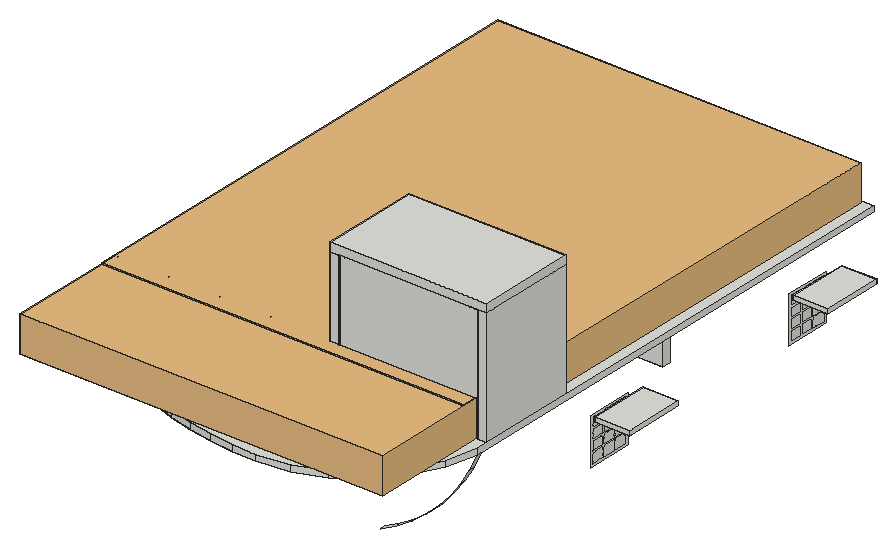
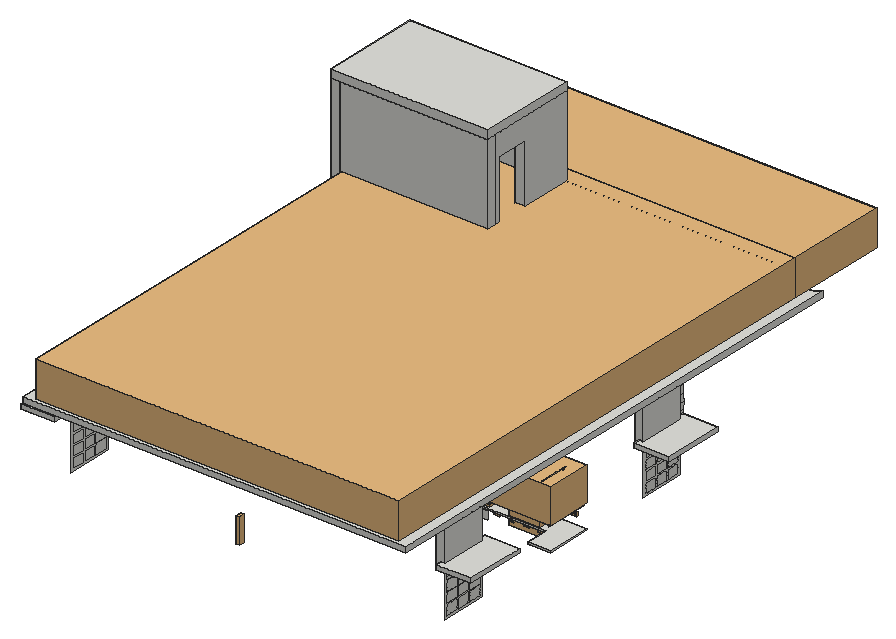
# SketchUp Ruby script. Lengths in inches.
U = 1.inch
M = Sketchup.active_model
def pt(a) = Geom::Point3d.new(a.map { |v| v * U })
def face(e, loops, mat)
  f = e.add_face(loops[0].map { |a| pt(a) })
  loops[1..].each { |l| e.add_face(l.map { |a| pt(a) }).erase! }
  f.material = f.back_material = mat if mat
  f
end
# faces: each face lists its corners as indices into pts; further lists are holes
def faces(e, pts, list, mat = nil) = list.each { |f| face(e, (f[0].is_a?(Array) ? f : [f]).map { |l| l.map { |i| pts[i] } }, mat) }
# xy, xz, yz: faces in a plane at the given z, y or x. An outline is a flat list of corners, or four numbers for a rectangle; further outlines are holes
def ring(l) = l.size == 4 ? [[l[0], l[1]], [l[2], l[1]], [l[2], l[3]], [l[0], l[3]]] : l.each_slice(2).to_a
def flat(e, list, mat, &to3) = list.each { |f| face(e, (f[0].is_a?(Array) ? f : [f]).map { |l| ring(l).map { |u, v| to3.(u, v) } }, mat) }
def xy(e, z, list, mat = nil) = flat(e, list, mat) { |x, y| [x, y, z] }
def xz(e, y, list, mat = nil) = flat(e, list, mat) { |x, z| [x, y, z] }
def yz(e, x, list, mat = nil) = flat(e, list, mat) { |y, z| [x, y, z] }
def lines(e, pts, list) = list.each { |a, b| e.add_line(pt(pts[a]), pt(pts[b])) }
# prism: a flat outline (further loops are holes) pulled along v
def prism(e, loops, v, mat = nil)
  f = face(e, loops, mat); d = Geom::Vector3d.new(v.map { |x| x * U })
  f.pushpull(f.normal.samedirection?(d) ? d.length : -d.length)
end
def box(e, o, s, mat = nil) = prism(e, [[o, [o[0] + s[0], o[1], o[2]], [o[0] + s[0], o[1] + s[1], o[2]], [o[0], o[1] + s[1], o[2]]]], [0, 0, s[2]], mat)
def at(x, y, z, deg = 0) = Geom::Transformation.translation(pt([x, y, z])) * Geom::Transformation.rotation(ORIGIN, Z_AXIS, deg.degrees)
def axes(o, x, y, z) = Geom::Transformation.new([*x, 0, *y, 0, *z, 0, *pt(o).to_a, 1])
def part(name) = M.definitions.add(name)
# library, detail: a bought-in or finely detailed component or shape, given as its bounding box
def library(name, o, s) = part(name).tap { |d| box(d.entities, o, s) }
def detail(e, o, s) = box(e.add_group.entities, o, s)
def put(e, d, t, mat = nil) = e.add_instance(d, t).tap { |i| i.material = mat if mat }
def group(e, t, mat = nil) = e.add_group.tap { |g| g.transformation = t; g.material = mat if mat }.entities
root = M.entities
c1 = library("00230906_3D_ducha_hig.dwg\#1",[121.96,-107.5,-116.36],[35.26,104.03,274.49])
c2 = part("Группа\#59")
xy(c2.entities,0,[[-13.1875,-4.13,13.1875,4.13]])
c3 = part("Panelled cabinet front \#2")
xy(c3.entities,0,[[[-15.55,-6.5,15.55,6.5],[-13.5,-4.45,13.5,4.45]]])
xy(c3.entities,0.98,[[[-15.55,-6.5,15.55,6.5],[-13.5,-4.45,13.5,4.45]]])
xz(c3.entities,-6.5,[[-15.55,0,15.55,0.98]])
xz(c3.entities,-4.13,[[-13.1875,0.31,13.1875,0.67]])
xz(c3.entities,4.13,[[-13.1875,0.31,13.1875,0.67]])
xz(c3.entities,6.5,[[-15.55,0,15.55,0.98]])
yz(c3.entities,-15.55,[[-6.5,0,6.5,0.98]])
yz(c3.entities,-13.1875,[[-4.13,0.31,4.13,0.67]])
yz(c3.entities,13.1875,[[-4.13,0.31,4.13,0.67]])
yz(c3.entities,15.55,[[-6.5,0,6.5,0.98]])
p = [[13.5,-4.45,0],[-13.5,-4.45,0],[13.1875,-4.13,0.31],[-13.1875,-4.13,0.31],[-13.1875,4.13,0.31],[-13.5,4.45,0],
  [13.1875,4.13,0.31],[13.5,4.45,0],[-13.5,4.45,0.98],[-13.5,-4.45,0.98],[-13.1875,-4.13,0.67],[13.5,-4.45,0.98],
  [13.1875,-4.13,0.67],[13.5,4.45,0.98],[-13.1875,4.13,0.67],[13.1875,4.13,0.67]]
faces(c3.entities,p,[[0,1,2],[3,2,1],[4,3,1],[1,5,4],[2,6,0],[0,6,7],[7,4,5],[6,4,7],
  [8,9,10],[11,10,9],[12,10,11],[11,13,12],[10,14,8],[15,12,13],[14,13,8],[14,15,13]])
put(c3.entities,c2,at(0,0,0.49))
c4 = part("Группа\#10")
xy(c4.entities,0,[[-13.1875,-4.13,13.1875,4.13]])
c5 = library("Gruppe\#5",[0,-1.9,0],[31.7,22.18,26.07])
c6 = part("Группа\#6")
prism(c6.entities,[[[-19.46,0,0],[-144,0,0],[-144,47.24,0],[-120.375,47.24,0],[-120.375,23.62,0],[-19.46,23.62,0]],[[-81.02,2.55,0],[-81.02,20.78,0],[-106.12,20.78,0],[-106.12,2.55,0]]],[0,0,1.57])
c7 = library("Group\#148",[0,0,0],[7.4375,14.82,1.97])
c8 = library("Group\#170",[0,0,0],[10.4375,12.4,1.97])
c9 = library("Group\#163",[0,0,0],[5.12,5.12,1.0625])
c10 = library("Group\#152",[0,0,0],[7.4375,14.82,1.97])
c11 = part("window_2")
xz(c11.entities,0,[[[-16,0,16,41],[-14,30.25,-5.25,39],[5.25,30.25,14,39],[5.25,2,14,10.75],[-14,2,-5.25,10.75],[-4.25,30.25,4.25,39],[-4.25,2,4.25,10.75],[5.25,21,14,29.25],[5.25,11.75,14,20],[-14,21,-5.25,29.25],[-14,11.75,-5.25,20],[-4.25,21,4.25,29.25],[-4.25,11.75,4.25,20]],[-14,2,-5.25,10.75],[-4.25,2,4.25,10.75],[5.25,2,14,10.75],[-14,11.75,-5.25,20],
  [-4.25,11.75,4.25,20],[5.25,11.75,14,20],[-14,21,-5.25,29.25],[-4.25,21,4.25,29.25],[5.25,21,14,29.25],
  [-14,30.25,-5.25,39],[-4.25,30.25,4.25,39],[5.25,30.25,14,39]])
c12 = library("Gruppe\#3",[0,0,0],[10.625,1.33,3.5625])
c13 = part("Component\#35")
detail(c13.entities,[0,0,0],[0.1,0.79,0.125])
c14 = library("Component\#38",[0,0,0],[0.16,0.16,0.04])
c15 = part("Группа\#7")
xz(c15.entities,1.5625,[[-122.05,-1.18,-77.55,0]])
p = [[-122.05,0,0],[-122.05,1.5625,0]]
lines(c15.entities,p,[[0,1]])
c16 = part("Группа\#121")
xz(c16.entities,0,[[[0,0,3.9375,3.9375],[0.39,0.39,3.54,3.54]]])
p = [[0.39,0,0.39],[1.97,0.39,1.97],[3.54,0,0.39],[0.39,0,3.54],[3.54,0,3.54]]
faces(c16.entities,p,[[0,1,2],[0,3,1],[4,2,1],[4,1,3]])
c17 = part("Группа\#14")
xy(c17.entities,0,[[0,-1.97,3.9375,9.84]])
xy(c17.entities,7.875,[[0,-1.97,3.9375,13.78]])
xz(c17.entities,-1.97,[[0,0,3.9375,7.875]])
yz(c17.entities,0,[[-1.97,0,-1.97,7.875,13.78,7.875,13.78,3.9375,13.3,3.81,12.84,3.65,12.4,3.4375,11.98,3.18,11.58,2.89,11.22,2.56,10.89,2.19,10.6,1.8,10.34,1.38,10.13,0.9375,9.96,0.48,9.84,0]])
yz(c17.entities,3.9375,[[-1.97,0,9.84,0,9.96,0.48,10.13,0.9375,10.34,1.38,10.6,1.8,10.89,2.19,11.22,2.56,11.58,2.89,11.98,3.18,12.4,3.4375,12.84,3.65,13.3,3.81,13.78,3.9375,13.78,7.875,-1.97,7.875]])
p = [[0,9.84,0],[0,9.96,0.48],[3.9375,9.96,0.48],[3.9375,9.84,0],[0,10.13,0.9375],[3.9375,10.13,0.9375],
  [0,10.34,1.38],[3.9375,10.34,1.38],[0,10.6,1.8],[3.9375,10.6,1.8],[0,10.89,2.19],[3.9375,10.89,2.19],
  [0,11.22,2.56],[3.9375,11.22,2.56],[0,11.58,2.89],[3.9375,11.58,2.89],[0,11.98,3.18],[3.9375,11.98,3.18],
  [0,12.4,3.4375],[3.9375,12.4,3.4375],[0,12.84,3.65],[3.9375,12.84,3.65],[0,13.3,3.81],[3.9375,13.3,3.81],
  [0,13.78,3.9375],[3.9375,13.78,3.9375]]
faces(c17.entities,p,[[0,1,2,3],[1,4,5,2],[4,6,7,5],[6,8,9,7],[8,10,11,9],[10,12,13,11],[12,14,15,13],[14,16,17,15],
  [16,18,19,17],[18,20,21,19],[20,22,23,21],[22,24,25,23]])
put(c17.entities,c16,at(0,13.78,3.9375))
c18 = part("Группа\#12")
xy(c18.entities,0,[[0,-1.97,3.9375,9.84]])
xy(c18.entities,7.875,[[0,-1.97,3.9375,13.78]])
xz(c18.entities,-1.97,[[0,0,3.9375,7.875]])
yz(c18.entities,0,[[-1.97,0,-1.97,7.875,13.78,7.875,13.78,3.9375,13.3,3.81,12.84,3.65,12.4,3.4375,11.98,3.18,11.58,2.89,11.22,2.56,10.89,2.19,10.6,1.8,10.34,1.38,10.13,0.9375,9.96,0.48,9.84,0]])
yz(c18.entities,3.9375,[[-1.97,0,9.84,0,9.96,0.48,10.13,0.9375,10.34,1.38,10.6,1.8,10.89,2.19,11.22,2.56,11.58,2.89,11.98,3.18,12.4,3.4375,12.84,3.65,13.3,3.81,13.78,3.9375,13.78,7.875,-1.97,7.875]])
p = [[0,9.84,0],[0,9.96,0.48],[3.9375,9.96,0.48],[3.9375,9.84,0],[0,10.13,0.9375],[3.9375,10.13,0.9375],
  [0,10.34,1.38],[3.9375,10.34,1.38],[0,10.6,1.8],[3.9375,10.6,1.8],[0,10.89,2.19],[3.9375,10.89,2.19],
  [0,11.22,2.56],[3.9375,11.22,2.56],[0,11.58,2.89],[3.9375,11.58,2.89],[0,11.98,3.18],[3.9375,11.98,3.18],
  [0,12.4,3.4375],[3.9375,12.4,3.4375],[0,12.84,3.65],[3.9375,12.84,3.65],[0,13.3,3.81],[3.9375,13.3,3.81],
  [0,13.78,3.9375],[3.9375,13.78,3.9375]]
faces(c18.entities,p,[[0,1,2,3],[1,4,5,2],[4,6,7,5],[6,8,9,7],[8,10,11,9],[10,12,13,11],[12,14,15,13],[14,16,17,15],
  [16,18,19,17],[18,20,21,19],[20,22,23,21],[22,24,25,23]])
put(c18.entities,c16,at(0,13.78,3.9375))
c19 = library("Группа\#11",[-9.65,-17.52,0],[19.3,35.04,0.98])
c20 = library("Группа\#2",[-9.65,-17.52,0],[19.3,35.04,0.98])
c21 = library("Группа\#17",[-11.61,-17.52,0],[23.22,35.04,0.98])
c22 = part("Группа\#9")
xy(c22.entities,0,[[[-5.71,-17.52,5.71,17.52],[-3.66,-15.47,3.66,15.47]]])
xy(c22.entities,0.49,[[-3.35,-15.16,3.35,15.16]])
xy(c22.entities,0.98,[[[-5.71,-17.52,5.71,17.52],[-3.66,-15.47,3.66,15.47]]])
xz(c22.entities,-17.52,[[-5.71,0,5.71,0.98]])
xz(c22.entities,-15.16,[[-3.35,0.31,3.35,0.49],[-3.35,0.49,3.35,0.67]])
xz(c22.entities,15.16,[[-3.35,0.31,3.35,0.49],[-3.35,0.49,3.35,0.67]])
xz(c22.entities,17.52,[[-5.71,0,5.71,0.98]])
yz(c22.entities,-5.71,[[-17.52,0,17.52,0.98]])
yz(c22.entities,-3.35,[[-15.16,0.31,15.16,0.49],[-15.16,0.49,15.16,0.67]])
yz(c22.entities,3.35,[[-15.16,0.31,15.16,0.49],[-15.16,0.49,15.16,0.67]])
yz(c22.entities,5.71,[[-17.52,0,17.52,0.98]])
p = [[-3.35,-15.16,0.31],[3.35,-15.16,0.31],[-3.66,-15.47,0],[-3.66,15.47,0],[3.66,-15.47,0],[3.35,15.16,0.31],
  [3.66,15.47,0],[-3.35,15.16,0.31],[-3.35,-15.16,0.67],[-3.35,15.16,0.67],[-3.66,-15.47,0.98],[3.66,-15.47,0.98],
  [-3.66,15.47,0.98],[3.35,-15.16,0.67],[3.35,15.16,0.67],[3.66,15.47,0.98]]
faces(c22.entities,p,[[0,1,2],[2,3,0],[2,1,4],[5,4,1],[6,4,5],[7,0,3],[3,6,7],[5,7,6],
  [8,9,10],[10,11,8],[10,9,12],[13,8,11],[14,13,11],[14,11,15],[15,12,9],[14,15,9]])
c23 = part("Группа\#16")
xy(c23.entities,0,[[[-5.51,-17.52,5.51,17.52],[-3.46,-15.47,3.46,15.47]]])
xy(c23.entities,0.49,[[-3.15,-15.16,3.15,15.16]])
xy(c23.entities,0.98,[[[-5.51,-17.52,5.51,17.52],[-3.46,-15.47,3.46,15.47]]])
xz(c23.entities,-17.52,[[-5.51,0,5.51,0.98]])
xz(c23.entities,-15.16,[[-3.15,0.31,3.15,0.49],[-3.15,0.49,3.15,0.67]])
xz(c23.entities,15.16,[[-3.15,0.31,3.15,0.49],[-3.15,0.49,3.15,0.67]])
xz(c23.entities,17.52,[[-5.51,0,5.51,0.98]])
yz(c23.entities,-5.51,[[-17.52,0,17.52,0.98]])
yz(c23.entities,-3.15,[[-15.16,0.31,15.16,0.49],[-15.16,0.49,15.16,0.67]])
yz(c23.entities,3.15,[[-15.16,0.31,15.16,0.49],[-15.16,0.49,15.16,0.67]])
yz(c23.entities,5.51,[[-17.52,0,17.52,0.98]])
p = [[-3.15,-15.16,0.31],[3.15,-15.16,0.31],[-3.46,-15.47,0],[-3.46,15.47,0],[3.46,-15.47,0],[3.15,15.16,0.31],
  [3.46,15.47,0],[-3.15,15.16,0.31],[-3.15,-15.16,0.67],[-3.15,15.16,0.67],[-3.46,-15.47,0.98],[3.46,-15.47,0.98],
  [-3.46,15.47,0.98],[3.15,-15.16,0.67],[3.15,15.16,0.67],[3.46,15.47,0.98]]
faces(c23.entities,p,[[0,1,2],[2,3,0],[2,1,4],[5,4,1],[6,4,5],[7,0,3],[3,6,7],[5,7,6],
  [8,9,10],[10,11,8],[10,9,12],[13,8,11],[14,13,11],[14,11,15],[15,12,9],[14,15,9]])
c24 = part("Группа\#4")
xy(c24.entities,0,[[-3.05,-15.16,3.05,15.16]])
c25 = part("Group\#14")
xy(c25.entities,36,[[0,0,9,48]])
yz(c25.entities,0,[[0,0,48,36]])
yz(c25.entities,9,[[0,0,48,36]])
c26 = part("Group\#17")
box(c26.entities,[0,0,0],[36,62.875,4.625])
c27 = library("Group\#4",[0,0,0],[375.02,122.21,36.98])
c28 = library("Group\#235",[0,0,0],[375.14,512.86,37.57])
prism(root,[[[52.638,387.274,167.253],[52.658,387.274,167.25],[52.679,387.274,167.253],[52.698,387.274,167.261],[52.714,387.274,167.273],[52.726,387.274,167.289],[52.734,387.274,167.308],[52.737,387.274,167.329],[52.734,387.274,167.349],[52.726,387.274,167.368],[52.714,387.274,167.384],[52.698,387.274,167.397],[52.679,387.274,167.405],[52.658,387.274,167.407],[52.638,387.274,167.405],[52.619,387.274,167.397],[52.602,387.274,167.384],[52.59,387.274,167.368],[52.582,387.274,167.349],[52.579,387.274,167.329],[52.582,387.274,167.308],[52.59,387.274,167.289],[52.602,387.274,167.273],[52.619,387.274,167.261]]],[0,-0.002,0])
prism(root,[[[56.178,387.274,167.263],[56.199,387.274,167.26],[56.219,387.274,167.263],[56.238,387.274,167.27],[56.254,387.274,167.283],[56.267,387.274,167.299],[56.275,387.274,167.318],[56.278,387.274,167.339],[56.275,387.274,167.359],[56.267,387.274,167.378],[56.254,387.274,167.394],[56.238,387.274,167.407],[56.219,387.274,167.415],[56.199,387.274,167.417],[56.178,387.274,167.415],[56.159,387.274,167.407],[56.143,387.274,167.394],[56.131,387.274,167.378],[56.123,387.274,167.359],[56.12,387.274,167.339],[56.123,387.274,167.318],[56.131,387.274,167.299],[56.143,387.274,167.283],[56.159,387.274,167.27]]],[0,-0.002,0])
prism(root,[[[59.739,387.272,167.27],[59.719,387.272,167.272],[59.7,387.272,167.28],[59.684,387.272,167.293],[59.671,387.272,167.309],[59.663,387.272,167.328],[59.661,387.272,167.348],[59.663,387.272,167.369],[59.671,387.272,167.388],[59.684,387.272,167.404],[59.7,387.272,167.417],[59.719,387.272,167.424],[59.739,387.272,167.427],[59.76,387.272,167.424],[59.779,387.272,167.417],[59.795,387.272,167.404],[59.808,387.272,167.388],[59.816,387.272,167.369],[59.818,387.272,167.348],[59.816,387.272,167.328],[59.808,387.272,167.309],[59.795,387.272,167.293],[59.779,387.272,167.28],[59.76,387.272,167.272]]],[0,0.002,0])
box(root,[428.25,528.25,210],[36,62.875,4.625])
box(root,[428.25,271.75,210],[36,62.875,4.625])
xy(root,152.378,[[109.514,386.793,109.675,386.814,109.825,386.876,109.954,386.975,110.052,387.104,110.115,387.254,110.136,387.415,110.115,387.576,110.052,387.726,109.954,387.855,109.825,387.954,109.675,388.016,109.514,388.037,109.353,388.016,109.203,387.954,109.074,387.855,108.975,387.726,108.913,387.576,108.892,387.415,108.913,387.254,108.975,387.104,109.074,386.975,109.203,386.876,109.353,386.814]])
xy(root,152.772,[[[109.514,386.628,109.718,386.654,109.908,386.733,110.071,386.858,110.196,387.021,110.274,387.211,110.301,387.415,110.274,387.619,110.196,387.809,110.071,387.972,109.908,388.097,109.718,388.176,109.514,388.202,109.31,388.176,109.12,388.097,108.957,387.972,108.832,387.809,108.753,387.619,108.726,387.415,108.753,387.211,108.832,387.021,108.957,386.858,109.12,386.733,109.31,386.654],[109.514,386.793,109.353,386.814,109.203,386.876,109.074,386.975,108.975,387.104,108.913,387.254,108.892,387.415,108.913,387.576,108.975,387.726,109.074,387.855,109.203,387.954,109.353,388.016,109.514,388.037,109.675,388.016,109.825,387.954,109.954,387.855,110.052,387.726,110.115,387.576,110.136,387.415,110.115,387.254,110.052,387.104,109.954,386.975,109.825,386.876,109.675,386.814]]])
xy(root,246,[[[295.125,0,327.528,3.982,358.004,15.69,384.738,34.428,406.141,59.081,420.938,88.182,428.25,120,257.25,120,257.25,129,428.25,129,428.25,633,32.25,633,32.25,93.378,34.093,94.889,36.109,96.159,38.268,97.168,40.536,97.9,42.877,98.344,45.256,98.493,47.634,98.344,49.976,97.9,52.243,97.168,54.402,96.159,56.419,94.889,58.262,93.378,67.349,84.921,86.685,69.348,107.082,55.192,128.437,42.528,150.64,31.419,173.579,21.921,197.137,14.083,221.194,7.945,245.628,3.539,270.313,0.886],[275.25,141.125,419.25,225],[72.5,219,99.9375,225]],[257.25,120,428.25,129],[72.5,219,99.9375,225]])
xy(root,252,[[[295.125,0,327.528,3.982,358.004,15.69,384.738,34.428,406.141,59.081,420.938,88.182,428.25,120,428.25,633,32.25,633,32.25,93.378,34.093,94.889,36.109,96.159,38.268,97.168,40.536,97.9,42.877,98.344,45.256,98.493,47.634,98.344,49.976,97.9,52.243,97.168,54.402,96.159,56.419,94.889,58.262,93.378,67.349,84.921,86.685,69.348,107.082,55.192,128.437,42.528,150.64,31.419,173.579,21.921,197.137,14.083,221.194,7.945,245.628,3.539,270.313,0.886],[294.589,12.365,271.194,13.201,247.384,15.759,223.818,20.01,200.615,25.93,177.892,33.489,155.767,42.65,134.352,53.365,113.755,65.58,94.082,79.233,75.432,94.254,66.384,102.673,63.647,104.918,60.325,107.01,56.768,108.673,53.032,109.879,49.174,110.61,45.256,110.855,44.588,110.813,44.588,620.662,415.912,620.662,415.912,234,419.25,234,419.25,141.125,415.912,141.125,415.912,121.399,409.253,92.423,395.83,66.025,376.415,43.661,352.164,26.664,324.519,16.043],[415.656,141.125,415.912,225]],[294.589,12.365,324.519,16.043,352.164,26.664,376.415,43.661,395.83,66.025,409.253,92.423,415.912,121.399,415.912,141.125,275.25,141.125,275.25,132.125,266.25,132.125,266.25,234,415.912,234,415.912,620.662,44.588,620.662,44.588,110.813,45.256,110.855,49.174,110.61,53.032,109.879,56.768,108.673,60.325,107.01,63.647,104.918,66.384,102.673,75.432,94.254,94.082,79.233,113.755,65.58,134.352,53.365,155.767,42.65,177.892,33.489,200.615,25.93,223.818,20.01,247.384,15.759,271.194,13.201],[415.656,141.125,415.912,225],[415.912,141.125,419.25,225],[266.25,225,415.656,234],
  [415.656,225,415.912,234],[415.912,225,419.25,234]])
xy(root,372,[[419.25,132.125,428.25,234],[266.25,225,419.25,234]])
xz(root,132.125,[[419.25,252,428.25,372]])
xz(root,225,[[266.25,252,419.25,372]])
xz(root,234,[[266.25,252,419.25,372],[419.25,252,428.25,372]])
xz(root,633,[[32.25,246,428.25,252]])
yz(root,32.25,[[93.378,246,633,252]])
yz(root,143.548,[[405.828,158.839,405.823,158.841,405.97,159.413,405.975,159.411],[405.823,158.841,404.574,159.161,404.721,159.733,405.97,159.413]])
yz(root,143.862,[[405.826,158.84,405.973,159.412,405.97,159.413,405.823,158.841],[405.823,158.841,405.97,159.413,404.717,159.734,404.57,159.162]])
yz(root,266.25,[[225,252,234,372]])
yz(root,419.25,[[132.125,252,225,372],[225,252,234,372]])
yz(root,428.25,[[120,246,633,252],[132.125,252,234,372]])
p = [[344.873,120,150.995],[328.466,120,142.687],[328.466,124.9375,142.687],[344.873,124.9375,150.995],[84.135,219,145.182],[84.135,223.125,145.182],
  [81.597,223.125,152.253],[81.597,219,152.253],[87.668,219,152.001],[87.668,223.125,152.001],[81.597,225,152.253],[84.135,225,145.182],
  [87.668,225,152.001],[360.414,120,160.829],[360.414,124.9375,160.829],[90.596,219,159.1],[90.596,223.125,159.1],[90.596,225,159.1],
  [79.506,223.125,159.47],[79.506,219,159.47],[79.506,225,159.47],[109.203,386.876,152.772],[109.353,386.814,152.772],[109.353,386.814,152.378],
  [109.203,386.876,152.378],[109.514,386.793,152.772],[109.514,386.793,152.378],[109.675,386.814,152.772],[109.675,386.814,152.378],[109.825,386.876,152.772],
  [109.825,386.876,152.378],[109.074,386.975,152.772],[109.074,386.975,152.378],[109.954,386.975,152.772],[109.954,386.975,152.378],[108.975,387.104,152.772],
  [108.975,387.104,152.378],[110.052,387.104,152.772],[110.052,387.104,152.378],[108.913,387.254,152.772],[108.913,387.254,152.378],[110.115,387.254,152.772],
  [110.115,387.254,152.378],[108.892,387.415,152.772],[108.892,387.415,152.378],[110.136,387.415,152.772],[110.136,387.415,152.378],[108.913,387.576,152.772],
  [108.913,387.576,152.378],[110.115,387.576,152.772],[110.115,387.576,152.378],[108.975,387.726,152.772],[108.975,387.726,152.378],[110.052,387.726,152.772],
  [110.052,387.726,152.378],[109.074,387.855,152.772],[109.074,387.855,152.378],[109.954,387.855,152.772],[109.954,387.855,152.378],[109.203,387.954,152.772],
  [109.203,387.954,152.378],[109.825,387.954,152.772],[109.825,387.954,152.378],[109.353,388.016,152.772],[109.353,388.016,152.378],[109.514,388.037,152.772],
  [109.514,388.037,152.378],[109.675,388.016,152.772],[109.675,388.016,152.378],[143.114,404.798,158.697],[143.054,404.957,158.657],[143.037,405.125,158.613],
  [143.066,405.292,158.571],[143.139,405.446,158.531],[143.25,405.577,158.498],[143.393,405.675,158.472],[143.557,405.734,158.457],[143.73,405.75,158.453],
  [143.903,405.721,158.46],[144.062,405.651,158.478],[144.196,405.543,158.506],[144.297,405.405,158.542],[144.358,405.246,158.582],[144.375,405.078,158.626],
  [144.346,404.911,158.668],[144.273,404.757,158.708],[144.162,404.627,158.741],[144.019,404.529,158.767],[143.855,404.47,158.782],[143.681,404.454,158.786],
  [143.509,404.482,158.779],[143.35,404.553,158.76],[143.216,404.66,158.733],[144.297,405.503,158.923],[144.358,405.344,158.964],[143.066,405.39,158.952],
  [143.139,405.544,158.912],[143.25,405.674,158.879],[144.196,405.641,158.887],[144.062,405.749,158.86],[143.393,405.773,158.854],[143.548,405.828,158.839],
  [143.557,405.832,158.839],[143.573,405.834,158.838],[143.573,405.98,159.41],[143.705,405.992,159.407],[143.705,405.845,158.835],[143.73,405.847,158.834],
  [143.758,405.843,158.836],[143.758,405.99,159.408],[143.862,405.973,159.412],[143.862,405.826,158.84],[143.903,405.819,158.842],[144.375,405.176,159.007],
  [144.346,405.009,159.05],[143.054,405.055,159.038],[143.037,405.223,158.995],[144.162,404.725,159.123],[144.019,404.627,159.148],[143.35,404.65,159.142],
  [143.216,404.758,159.114],[144.273,404.855,159.089],[143.114,404.896,159.079],[143.509,404.58,159.16],[143.681,404.552,159.167],[143.652,404.557,159.166],
  [143.652,404.703,159.738],[143.548,404.721,159.733],[143.548,404.574,159.161],[143.855,404.568,159.163],[143.837,404.565,159.164],[143.837,404.712,159.736],
  [143.705,404.701,159.739],[143.705,404.554,159.167],[143.862,404.57,159.162],[143.548,405.823,158.841],[143.862,405.823,158.841],[143.548,405.975,159.411],
  [143.732,405.844,158.835],[143.732,405.991,159.407],[92.897,219,166.427],[92.897,223.125,166.427],[92.897,225,166.427],[143.678,404.555,159.166],
  [143.678,404.702,159.738],[143.862,404.717,159.734],[143.548,405.97,159.413],[143.862,405.97,159.413],[77.872,223.125,166.803],[77.872,219,166.803],
  [77.872,225,166.803],[374.946,120,172.1],[374.946,124.9375,172.1],[94.552,219,173.926],[94.552,223.125,173.926],[94.552,225,173.926],
  [76.7,223.125,174.224],[76.7,219,174.224],[76.7,225,174.224],[388.339,120,184.703],[388.339,124.9375,184.703],[95.551,219,181.541],
  [95.551,223.125,181.541],[95.551,225,181.541],[75.995,223.125,181.704],[75.995,219,181.704],[75.995,225,181.704],[95.885,219,189.213],
  [95.885,223.125,189.213],[95.885,225,189.213],[75.76,223.125,189.213],[75.76,219,189.213],[75.76,225,189.213],[400.47,120,198.526],
  [400.47,124.9375,198.526],[75.995,223.125,196.723],[75.995,219,196.723],[95.551,219,196.886],[95.551,223.125,196.886],[75.995,225,196.723],
  [95.551,225,196.886],[76.7,223.125,204.203],[76.7,219,204.203],[76.7,225,204.203],[94.552,219,204.5],[94.552,223.125,204.5],
  [94.552,225,204.5],[411.228,120,213.441],[411.228,124.9375,213.441],[77.872,223.125,211.624],[77.872,219,211.624],[77.872,225,211.624],
  [92.897,219,211.999],[92.897,223.125,211.999],[92.897,225,211.999],[79.506,223.125,218.957],[79.506,219,218.957],[79.506,225,218.957],
  [90.596,219,219.326],[90.596,223.125,219.326],[90.596,225,219.326],[420.517,120,229.314],[420.517,124.9375,229.314],[81.597,223.125,226.173],
  [81.597,219,226.173],[81.597,225,226.173],[87.668,219,226.426],[87.668,223.125,226.426],[87.668,225,226.426],[84.135,223.125,233.245],
  [84.135,219,233.245],[84.135,225,233.245],[428.25,120,246],[428.25,124.9375,246],[295.125,0,252],[270.313,0.886,252],
  [270.313,0.886,246],[295.125,0,246],[327.528,3.982,252],[327.528,3.982,246],[245.628,3.539,252],[245.628,3.539,246],
  [221.194,7.945,252],[221.194,7.945,246],[358.004,15.69,252],[358.004,15.69,246],[197.137,14.083,252],[197.137,14.083,246],
  [173.579,21.921,252],[173.579,21.921,246],[384.738,34.428,252],[384.738,34.428,246],[150.64,31.419,252],[150.64,31.419,246],
  [128.437,42.528,252],[128.437,42.528,246],[406.141,59.081,252],[406.141,59.081,246],[107.082,55.192,252],[107.082,55.192,246],
  [86.685,69.348,252],[86.685,69.348,246],[420.938,88.182,252],[420.938,88.182,246],[67.349,84.921,252],[67.349,84.921,246],
  [58.262,93.378,252],[58.262,93.378,246],[428.25,120,252],[34.093,94.889,252],[32.25,93.378,252],[32.25,93.378,246],
  [34.093,94.889,246],[56.419,94.889,252],[56.419,94.889,246],[36.109,96.159,252],[36.109,96.159,246],[54.402,96.159,252],
  [54.402,96.159,246],[38.268,97.168,252],[38.268,97.168,246],[52.243,97.168,252],[52.243,97.168,246],[40.536,97.9,252],
  [40.536,97.9,246],[49.976,97.9,252],[49.976,97.9,246],[42.877,98.344,252],[42.877,98.344,246],[47.634,98.344,252],
  [47.634,98.344,246],[45.256,98.493,252],[45.256,98.493,246],[52.698,387.276,167.397],[52.698,387.274,167.397],[52.602,387.276,167.384],
  [52.602,387.274,167.384],[52.679,387.276,167.253],[52.679,387.274,167.253],[52.59,387.276,167.289],[52.59,387.274,167.289],[52.698,387.276,167.261],
  [52.698,387.274,167.261],[52.726,387.276,167.368],[52.726,387.274,167.368],[52.619,387.276,167.261],[52.619,387.274,167.261],[52.602,387.276,167.273],
  [52.602,387.274,167.273],[52.734,387.276,167.308],[52.734,387.274,167.308],[52.726,387.276,167.289],[52.726,387.274,167.289],[52.714,387.276,167.273],
  [52.714,387.274,167.273],[52.734,387.276,167.349],[52.734,387.274,167.349],[52.737,387.276,167.329],[52.737,387.274,167.329],[52.638,387.276,167.253],
  [52.638,387.274,167.253],[52.638,387.276,167.405],[52.638,387.274,167.405],[52.658,387.276,167.25],[52.658,387.274,167.25],[52.579,387.276,167.329],
  [52.579,387.274,167.329],[52.619,387.276,167.397],[52.619,387.274,167.397],[52.658,387.276,167.407],[52.658,387.274,167.407],[52.714,387.276,167.384],
  [52.714,387.274,167.384],[52.679,387.276,167.405],[52.679,387.274,167.405],[52.582,387.276,167.308],[52.582,387.274,167.308],[52.59,387.276,167.368],
  [52.59,387.274,167.368],[52.582,387.276,167.349],[52.582,387.274,167.349],[53.061,410.819,181.315],[53.061,434.047,181.315],[163.511,398.811,216.551],
  [163.441,399.06,216.551],[143.548,404.565,159.164],[143.81,404.561,159.165],[143.784,404.558,159.166],[143.758,404.555,159.166],[143.731,404.554,159.167],
  [56.159,387.276,167.407],[56.159,387.274,167.407],[56.275,387.276,167.318],[56.275,387.274,167.318],[56.131,387.276,167.378],[56.131,387.274,167.378],
  [56.199,387.276,167.417],[56.199,387.274,167.417],[56.219,387.276,167.263],[56.219,387.274,167.263],[56.238,387.276,167.407],[56.238,387.274,167.407],
  [56.254,387.276,167.283],[56.254,387.274,167.283],[153.59,405.961,158.48],[153.588,405.882,158.48],[56.123,387.276,167.359],[56.123,387.274,167.359],
  [143.599,404.563,159.164],[143.573,404.568,159.163],[143.626,404.559,159.165],[136.092,405.838,158.837],[136.068,405.841,158.836],[56.143,387.276,167.394],
  [56.143,387.274,167.394],[56.267,387.276,167.378],[56.267,387.274,167.378],[56.159,387.276,167.27],[56.159,387.274,167.27],[56.143,387.276,167.283],
  [56.143,387.274,167.283],[56.238,387.276,167.27],[56.238,387.274,167.27],[56.178,387.276,167.263],[56.178,387.274,167.263],[56.12,387.276,167.339],
  [56.12,387.274,167.339],[56.267,387.276,167.299],[56.267,387.274,167.299],[56.178,387.276,167.415],[56.178,387.274,167.415],[56.199,387.276,167.26],
  [56.199,387.274,167.26],[56.254,387.276,167.394],[56.254,387.274,167.394],[56.219,387.276,167.415],[56.219,387.274,167.415],[56.278,387.276,167.339],
  [56.278,387.274,167.339],[56.275,387.276,167.359],[56.275,387.274,167.359],[56.131,387.276,167.299],[56.131,387.274,167.299],[56.123,387.276,167.318],
  [56.123,387.274,167.318],[53.061,410.819,216.354],[53.061,434.047,216.354],[199.25,225,209.373],[236.927,225,209.373],[236.927,225,246],
  [41.25,624,246],[32.25,624,246],[199.25,225,246],[59.808,387.276,167.388],[59.808,387.274,167.388],[59.816,387.276,167.328],
  [59.816,387.274,167.328],[59.671,387.276,167.388],[59.671,387.274,167.388],[59.816,387.276,167.369],[59.816,387.274,167.369],[59.795,387.276,167.293],
  [59.795,387.274,167.293],[59.661,387.276,167.348],[59.661,387.274,167.348],[59.663,387.276,167.369],[59.663,387.274,167.369],[59.684,387.276,167.404],
  [59.684,387.274,167.404],[59.818,387.276,167.348],[59.818,387.274,167.348],[59.7,387.276,167.28],[59.7,387.274,167.28],[59.795,387.276,167.404],
  [59.795,387.274,167.404],[59.739,387.276,167.427],[59.739,387.274,167.427],[59.663,387.276,167.328],[59.663,387.274,167.328],[59.779,387.276,167.417],
  [59.779,387.274,167.417],[59.719,387.276,167.272],[59.719,387.274,167.272],[59.76,387.276,167.424],[59.76,387.274,167.424],[59.671,387.276,167.309],
  [59.671,387.274,167.309],[59.7,387.276,167.417],[59.7,387.274,167.417],[59.808,387.276,167.309],[59.808,387.274,167.309],[59.719,387.276,167.424],
  [59.719,387.274,167.424],[59.684,387.276,167.293],[59.684,387.274,167.293],[59.76,387.276,167.272],[59.76,387.274,167.272],[59.779,387.276,167.28],
  [59.779,387.274,167.28],[59.739,387.276,167.27],[59.739,387.274,167.27],[143.652,405.844,158.835],[143.626,405.841,158.836],[143.679,405.845,158.835],
  [143.6,405.838,158.837],[143.811,405.836,158.837],[143.784,405.84,158.836],[143.837,405.832,158.839],[137.998,405.841,158.836],[137.971,405.843,158.836],
  [138.024,405.837,158.837],[137.945,405.844,158.835],[137.918,405.844,158.835],[136.246,404.507,158.772],[136.396,404.59,158.751],[135.594,405.613,158.488],
  [135.471,405.495,158.518],[135.384,405.351,158.556],[136.042,405.843,158.836],[136.519,404.708,158.721],[136.606,404.853,158.683],[135.912,405.739,158.456],
  [135.745,405.696,158.467],[136.609,405.344,158.557],[136.523,405.49,158.52],[136.402,405.609,158.489],[136.252,405.694,158.467],[136.652,405.015,158.642],
  [136.016,405.844,158.835],[135.989,405.844,158.835],[136.078,404.464,158.783],[135.337,405.021,158.64],[135.381,404.859,158.682],[143.862,404.565,159.164],
  [136.085,405.738,158.456],[135.738,404.51,158.771],[135.905,404.465,158.783],[135.338,405.189,158.597],[135.589,404.594,158.75],[135.467,404.713,158.719],
  [136.653,405.182,158.599],[43.662,627.811,252.591],[43.662,118.491,252.591],[415.656,620.406,252],[415.656,234,252],[266.25,132.125,372],
  [419.25,132.125,372],[266.25,225,372]]
faces(root,p,[[0,1,2,3],[4,5,6,7],[8,9,5,4],[10,6,5,11],[11,5,9,12],[13,0,3,14],[15,16,9,8],[12,9,16,17],
  [7,6,18,19],[20,18,6,10],[21,22,23,24],[22,25,26,23],[25,27,28,26],[27,29,30,28],[31,21,24,32],[29,33,34,30],
  [35,31,32,36],[33,37,38,34],[39,35,36,40],[37,41,42,38],[43,39,40,44],[41,45,46,42],[47,43,44,48],[45,49,50,46],
  [51,47,48,52],[49,53,54,50],[55,51,52,56],[53,57,58,54],[59,55,56,60],[57,61,62,58],[63,59,60,64],[65,63,64,66],
  [67,65,66,68],[61,67,68,62],[69,70,71,72,73,74,75,76,77,78,79,80,81,82,83,84,85,86,87,88,89,90,91,92],[82,81,93,94],[73,72,95,96],[74,73,96,97],[81,80,98,93],[80,79,99,98],
  [75,74,97,100],[76,75,100,101,102],[77,76,102,103,104,105,106,107],[78,77,107,108,109,110,111,112],[79,78,112,99],[84,83,113,114],[71,70,115,116],[72,71,116,95],
  [83,82,94,113],[87,86,117,118],[92,91,119,120],[86,85,121,117],[69,92,120,122],[70,69,122,115],[85,84,114,121],[91,90,123,119],
  [90,89,124,125,126,127,128,123],[89,88,129,130,131,132,133,124],[88,87,118,134,129],[123,128,135,101,100,97,96,95,116,115,122,120,119],[112,111,136,134,118,117,121,114,113,94,93,98,99],[103,101,137,104],[138,106,105,139],[108,138,139,109],
  [140,141,16,15],[17,16,141,142],[143,133,132,144],[125,143,144,126],[130,134,145,131],[110,109,139,105,104,137,146,127,126,144,132,131,145,147],[19,18,148,149],[150,148,18,20],
  [151,13,14,152],[153,154,141,140],[142,141,154,155],[149,148,156,157],[158,156,148,150],[159,151,152,160],[161,162,154,153],[155,154,162,163],
  [157,156,164,165],[166,164,156,158],[167,168,162,161],[163,162,168,169],[165,164,170,171],[172,170,164,166],[173,159,160,174],[171,170,175,176],
  [177,178,168,167],[179,175,170,172],[169,168,178,180],[176,175,181,182],[183,181,175,179],[184,185,178,177],[180,178,185,186],[187,173,174,188],
  [182,181,189,190],[191,189,181,183],[192,193,185,184],[186,185,193,194],[190,189,195,196],[197,195,189,191],[198,199,193,192],[194,193,199,200],
  [201,187,188,202],[196,195,203,204],[205,203,195,197],[206,207,199,198],[200,199,207,208],[204,203,209,210],[211,209,203,205],[210,209,207,206],
  [208,207,209,211],[212,201,202,213],[214,215,216,217],[218,214,217,219],[215,220,221,216],[220,222,223,221],[224,218,219,225],[222,226,227,223],
  [226,228,229,227],[230,224,225,231],[228,232,233,229],[232,234,235,233],[236,230,231,237],[234,238,239,235],[238,240,241,239],[242,236,237,243],
  [240,244,245,241],[244,246,247,245],[248,242,243,212],[249,250,251,252],[246,253,254,247],[255,249,252,256],[253,257,258,254],[259,255,256,260],
  [257,261,262,258],[263,259,260,264],[261,265,266,262],[267,263,264,268],[265,269,270,266],[271,267,268,272],[269,271,272,270]])
lines(root,p,[[273,274],[275,276],[277,278],[279,280],[281,282],[283,284],[285,286],[287,288],[289,290],[291,292],[293,294],[295,296],
  [297,298],[299,300],[301,302],[303,304],[305,306],[307,308],[309,310],[311,312],[313,314],[315,316],[317,318],[319,320],
  [321,322],[323,324],[325,128],[130,326],[326,327],[327,328],[328,329],[329,133],[330,331],[332,333],[334,335],[336,337],
  [338,339],[340,341],[342,343],[344,345],[346,347],[348,349],[125,350],[350,348],[349,128],[351,352],[353,354],[355,356],
  [357,358],[359,360],[361,362],[363,364],[365,366],[367,368],[369,370],[371,372],[373,374],[375,376],[377,378],[379,380],
  [381,382],[383,384],[385,321],[386,385],[387,388],[388,389],[390,391],[322,386],[392,387],[393,394],[395,396],[397,398],
  [399,400],[401,402],[403,404],[405,406],[407,408],[409,410],[411,412],[413,414],[415,416],[417,418],[419,420],[421,422],
  [423,424],[425,426],[427,428],[429,430],[431,432],[433,434],[435,436],[437,438],[439,440],[441,442],[106,443],[443,441],
  [442,444],[444,103],[445,446],[111,447],[447,445],[446,108],[448,449],[450,448],[449,451],[451,452],[453,454],[455,456],
  [456,457],[352,458],[459,460],[461,462],[463,464],[465,466],[460,467],[458,468],[462,455],[468,469],[470,453],[471,472],
  [134,473],[466,474],[454,459],[475,476],[457,477],[478,475],[474,461],[479,478],[476,470],[464,465],[477,471],[480,463],
  [467,480],[472,479],[481,482],[483,481],[484,483],[485,486],[487,485]])
detail(root,[168.23,409.44,140.6],[5.89,1.12,1.51])
detail(root,[97.58,409.44,153.85],[5.89,1.12,1.51])
detail(root,[81.83,409.44,153.85],[5.89,1.12,1.51])
detail(root,[112.84,409.44,153.86],[5.89,1.12,1.52])
detail(root,[67.18,409.44,153.97],[5.89,1.12,1.51])
detail(root,[168.23,409.44,153.98],[5.89,1.12,1.52])
detail(root,[63.69,425.39,153.98],[1.12,5.89,1.52])
detail(root,[124.77,389.74,157.5],[30.2,18.11,1.77])
detail(root,[137.26,404.46,158.45],[1.33,1.53,1.29])
detail(root,[135.33,404.46,158.45],[1.33,1.53,1.29])
detail(root,[141.11,404.46,158.45],[1.33,1.53,1.29])
detail(root,[139.18,404.46,158.45],[1.33,1.53,1.29])
detail(root,[50.89,386.02,165.56],[10.62,1.29,3.56])
detail(root,[51.63,387.22,166.31],[2.05,0.13,2.04])
detail(root,[55.17,387.22,166.31],[2.05,0.13,2.05])
detail(root,[58.71,387.22,166.32],[2.05,0.13,2.05])
detail(root,[41.25,387,181.12],[122.55,47.24,35.43])
detail(root,[96.99,399.52,181.78],[1.27,1.56,1.27])
detail(root,[94.48,399.52,181.78],[1.27,1.56,1.27])
detail(root,[74.68,399.52,181.91],[1.27,1.56,1.27])
detail(root,[53.77,411.36,181.95],[1.56,1.28,1.28])
put(root,c1,axes([277.76,553.51,151.14],[-0.09516,0,0.0006],[0,-0.05567,-0.00034],[0.0006,-0.00058,0.09516]))
put(root,c3,axes([171.17,408.46,149.23],[-1,0,0],[0,0,1],[0,1,0]))
put(root,c4,axes([139.68,408.95,149.23],[-1,0,0],[0,0,1],[0,1,0]))
put(root,c5,at(72.53,388.57,148.6))
put(root,c6,at(185.25,387,155.92))
put(root,c7,axes([153.3125,391.39,160.17],[-1,0,0],[0,1,0],[0,0,-1]))
put(root,c8,axes([134.65,403.8,160.17],[1,0,0],[0,-1,0],[0,0,-1]))
put(root,c9,at(142.43,399.58,158.2,180))
put(root,c10,axes([126.42,406.21,160.17],[1,0,0],[0,-1,0],[0,0,-1]))
put(root,c11,axes([32.25,301.5,162],[0,-1.5,0],[1.17,0,0],[0,0,1.17]))
put(root,c11,axes([153.75,225,162],[1.5,0,0],[0,1.17,0],[0,0,1.17]))
put(root,c11,axes([32.25,558,162],[0,-1.5,0],[1.17,0,0],[0,0,1.17]))
put(root,c11,axes([419.25,558,162],[0,-1.5,0],[1.17,0,0],[0,0,1.17]))
put(root,c11,axes([419.25,301.5,162],[0,-1.5,0],[1.17,0,0],[0,0,1.17]))
put(root,c12,at(181.34,387.35,165.56,180))
put(root,c13,axes([52.71,387.34,166.61],[-1,0,0],[0,-0.11,0],[0,0,-1]))
put(root,c13,axes([56.25,387.34,166.62],[-1,0,0],[0,-0.11,0],[0,0,-1]))
put(root,c13,axes([59.79,387.34,166.63],[-1,0,0],[0,-0.11,0],[0,0,-1]))
put(root,c14,axes([52.74,387.27,167.25],[-1,0,0],[0,0,1],[0,0.11,0]))
put(root,c14,axes([56.28,387.27,167.26],[-1,0,0],[0,0,1],[0,0.11,0]))
put(root,c14,axes([59.82,387.27,167.27],[-1,0,0],[0,0,1],[0,0.11,0]))
put(root,c13,axes([52.71,387.34,168.05],[-1,0,0],[0,-0.11,0],[0,0,1]))
put(root,c13,axes([56.25,387.34,168.06],[-1,0,0],[0,-0.11,0],[0,0,1]))
put(root,c13,axes([59.79,387.34,168.07],[-1,0,0],[0,-0.11,0],[0,0,1]))
put(root,c15,at(40.71,312.33,181.12,-90))
put(root,c17,at(158.18,387.79,181.12))
put(root,c18,at(117.23,387.79,181.12))
put(root,c19,axes([106.21,398.54,198.83],[1,0,0],[0,0,1],[0,1,0]))
put(root,c20,axes([86.53,398.54,198.83],[-1,0,0],[0,0,1],[0,1,0]))
put(root,c21,axes([52.79,422.43,198.83],[0,1,0],[0,0,1],[1,0,0]))
put(root,c22,axes([70.78,398.54,198.83],[-1,0,0],[0,0,1],[0,1,0]))
put(root,c23,axes([52.79,405.13,198.83],[0,0.96,0],[0,0,1],[1,0,0]))
put(root,c24,axes([59.26,399.03,198.83],[-1,0,0],[0,0,1],[0,1,0]))
g1 = group(root,at(185.25,529.3125,209.375))
box(g1,[0,-37.3125,0],[9,37.3125,36.625])
g2 = group(root,at(414.25,387,209.375))
box(g2,[-34.5,-9,0],[34.5,9,36.625])
g3 = group(root,at(185.25,478,209.375))
box(g3,[0,-37.3125,0],[9,37.3125,36.625])
g4 = group(root,at(266.25,373.5,209.375,-90))
box(g4,[0,0,0],[37.68,9,36.625])
g5 = group(root,at(199.58,378,209.375))
box(g5,[0,0,0],[37.68,9,36.625])
g6 = group(root,at(199.25,225,209.375))
box(g6,[0,0,0],[37.68,9,36.625])
g7 = group(root,at(32.25,534,210))
xy(g7,0,[[0,0,9,48]])
xz(g7,0,[[0,0,9,36]])
xz(g7,48,[[0,0,9,36]])
put(g7,c25,at(0,0,0))
g8 = group(root,at(32.25,277.5,210))
xy(g8,0,[[0,0,9,48]])
xz(g8,0,[[0,0,9,36]])
xz(g8,48,[[0,0,9,36]])
put(g8,c25,at(0,0,0))
g9 = group(root,at(177.75,225,210,90))
xy(g9,0,[[0,0,9,48]])
xz(g9,0,[[0,0,9,36]])
xz(g9,48,[[0,0,9,36]])
put(g9,c25,at(0,0,0))
put(root,c26,at(0,525.84,210))
put(root,c26,at(0,269.34,210))
put(root,c27,at(42.47,11.02,252))
g10 = group(root,at(275.25,132.125,252))
box(g10,[0,0,0],[144,9,120])
put(root,c28,at(42.09,116.52,252))
g11 = group(root,at(266.25,132.125,252))
prism(g11,[[[0,92.875,0],[0,88.14,0],[0,88.14,97.9375],[0,53.875,97.9375],[0,53.875,0],[0,0,0],[0,0,120],[0,92.875,120]]],[10,0,0])
g12 = group(root,at(266.25,132.125,372))
xy(g12,0,[[0,0,162,101.875]])
xz(g12,0,[[0,0,162,9]])
xz(g12,101.875,[[0,0,162,9]])
yz(g12,0,[[0,0,101.875,9]])
yz(g12,162,[[0,0,101.875,9]])
g13 = group(g12,at(0,0,9))
xy(g13,0,[[0,0,162,101.875]])
